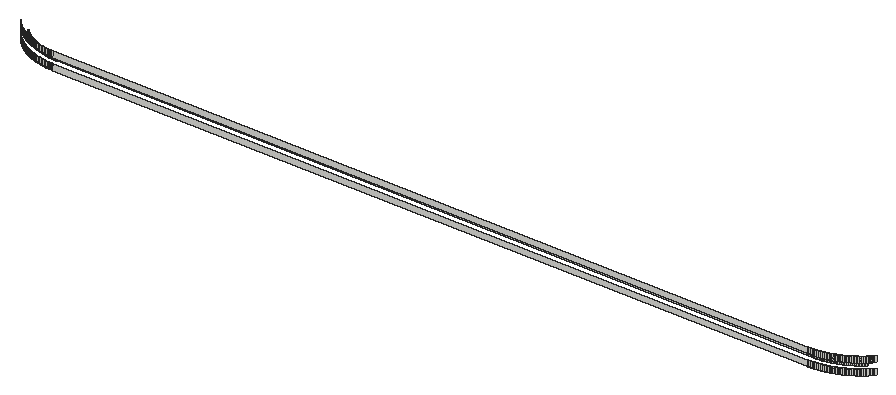
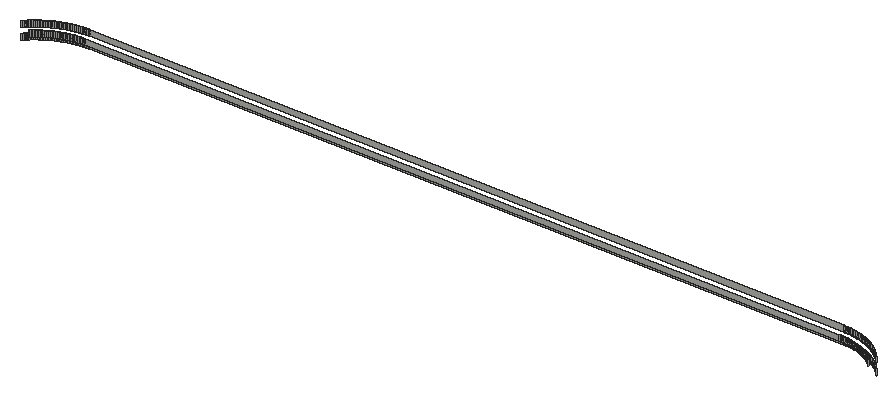
# SketchUp Ruby script. Lengths in inches.
U = 1.inch
M = Sketchup.active_model
def pt(a) = Geom::Point3d.new(a.map { |v| v * U })
def face(e, loops, mat)
  f = e.add_face(loops[0].map { |a| pt(a) })
  loops[1..].each { |l| e.add_face(l.map { |a| pt(a) }).erase! }
  f.material = f.back_material = mat if mat
  f
end
# faces: each face lists its corners as indices into pts; further lists are holes
def faces(e, pts, list, mat = nil) = list.each { |f| face(e, (f[0].is_a?(Array) ? f : [f]).map { |l| l.map { |i| pts[i] } }, mat) }
# xy, xz, yz: faces in a plane at the given z, y or x. An outline is a flat list of corners, or four numbers for a rectangle; further outlines are holes
def ring(l) = l.size == 4 ? [[l[0], l[1]], [l[2], l[1]], [l[2], l[3]], [l[0], l[3]]] : l.each_slice(2).to_a
def flat(e, list, mat, &to3) = list.each { |f| face(e, (f[0].is_a?(Array) ? f : [f]).map { |l| ring(l).map { |u, v| to3.(u, v) } }, mat) }
def xy(e, z, list, mat = nil) = flat(e, list, mat) { |x, y| [x, y, z] }
def xz(e, y, list, mat = nil) = flat(e, list, mat) { |x, z| [x, y, z] }
def yz(e, x, list, mat = nil) = flat(e, list, mat) { |y, z| [x, y, z] }
def lines(e, pts, list) = list.each { |a, b| e.add_line(pt(pts[a]), pt(pts[b])) }
# prism: a flat outline (further loops are holes) pulled along v
def prism(e, loops, v, mat = nil)
  f = face(e, loops, mat); d = Geom::Vector3d.new(v.map { |x| x * U })
  f.pushpull(f.normal.samedirection?(d) ? d.length : -d.length)
end
def box(e, o, s, mat = nil) = prism(e, [[o, [o[0] + s[0], o[1], o[2]], [o[0] + s[0], o[1] + s[1], o[2]], [o[0], o[1] + s[1], o[2]]]], [0, 0, s[2]], mat)
def at(x, y, z, deg = 0) = Geom::Transformation.translation(pt([x, y, z])) * Geom::Transformation.rotation(ORIGIN, Z_AXIS, deg.degrees)
def axes(o, x, y, z) = Geom::Transformation.new([*x, 0, *y, 0, *z, 0, *pt(o).to_a, 1])
def part(name) = M.definitions.add(name)
# library, detail: a bought-in or finely detailed component or shape, given as its bounding box
def library(name, o, s) = part(name).tap { |d| box(d.entities, o, s) }
def detail(e, o, s) = box(e.add_group.entities, o, s)
def put(e, d, t, mat = nil) = e.add_instance(d, t).tap { |i| i.material = mat if mat }
def group(e, t, mat = nil) = e.add_group.tap { |g| g.transformation = t; g.material = mat if mat }.entities
root = M.entities
xz(root,144,[[25.72,392.81,26.03,394.81],[26.03,392.81,290.42,394.81],[290.42,392.81,290.73,394.81],[25.72,396.81,26.03,398.81],[26.03,396.81,290.42,398.81],
  [290.42,396.81,290.73,398.81]])
xz(root,146,[[25.75,394.81,26.04,396.81],[26.04,394.81,290.41,396.81],[290.41,394.81,290.71,396.81]])
p = [[24.46,144.05,392.81],[24.78,144.03,392.81],[24.78,144.03,394.81],[24.46,144.05,394.81],[25.09,144.02,392.81],[25.09,144.02,394.81],
  [25.41,144.01,392.81],[25.41,144.01,394.81],[25.72,144,392.81],[25.72,144,394.81],[290.73,144,392.81],[291.05,144.01,392.81],
  [291.05,144.01,394.81],[290.73,144,394.81],[291.36,144.02,392.81],[291.36,144.02,394.81],[291.68,144.03,392.81],[291.68,144.03,394.81],
  [291.99,144.05,392.81],[291.99,144.05,394.81],[23.21,144.17,392.81],[23.52,144.13,392.81],[23.52,144.13,394.81],[23.21,144.17,394.81],
  [23.84,144.1,392.81],[23.84,144.1,394.81],[24.15,144.07,392.81],[24.15,144.07,394.81],[292.3,144.07,392.81],[292.3,144.07,394.81],
  [292.62,144.1,392.81],[292.62,144.1,394.81],[292.93,144.13,392.81],[292.93,144.13,394.81],[293.24,144.17,392.81],[293.24,144.17,394.81],
  [22.27,144.29,392.81],[22.59,144.25,392.81],[22.59,144.25,394.81],[22.27,144.29,394.81],[22.9,144.2,392.81],[22.9,144.2,394.81],
  [293.56,144.2,392.81],[293.56,144.2,394.81],[293.87,144.25,392.81],[293.87,144.25,394.81],[294.18,144.29,392.81],[294.18,144.29,394.81],
  [21.65,144.4,392.81],[21.96,144.35,392.81],[21.96,144.35,394.81],[21.65,144.4,394.81],[294.49,144.35,392.81],[294.49,144.35,394.81],
  [294.8,144.4,392.81],[294.8,144.4,394.81],[21.35,144.46,392.81],[21.35,144.46,394.81],[295.11,144.46,392.81],[295.11,144.46,394.81],
  [20.73,144.59,392.81],[21.04,144.52,392.81],[21.04,144.52,394.81],[20.73,144.59,394.81],[295.42,144.52,392.81],[295.42,144.52,394.81],
  [295.72,144.59,392.81],[295.72,144.59,394.81],[20.42,144.66,392.81],[20.42,144.66,394.81],[296.03,144.66,392.81],[296.03,144.66,394.81],
  [19.8125,144.82,392.81],[20.12,144.74,392.81],[20.12,144.74,394.81],[19.8125,144.82,394.81],[296.33,144.74,392.81],[296.33,144.74,394.81],
  [296.64,144.82,392.81],[296.64,144.82,394.81],[19.51,144.9,392.81],[19.51,144.9,394.81],[296.94,144.9,392.81],[296.94,144.9,394.81],
  [19.21,144.99,392.81],[19.21,144.99,394.81],[297.24,144.99,392.81],[297.24,144.99,394.81],[18.91,145.08,392.81],[18.91,145.08,394.81],
  [297.55,145.08,392.81],[297.55,145.08,394.81],[18.61,145.17,392.81],[18.61,145.17,394.81],[297.85,145.17,392.81],[297.85,145.17,394.81],
  [18.31,145.27,392.81],[18.31,145.27,394.81],[298.14,145.27,392.81],[298.14,145.27,394.81],[18.01,145.375,392.81],[18.01,145.375,394.81],
  [298.44,145.375,392.81],[298.44,145.375,394.81],[17.72,145.48,392.81],[17.72,145.48,394.81],[298.74,145.48,392.81],[298.74,145.48,394.81],
  [17.42,145.59,392.81],[17.42,145.59,394.81],[299.03,145.59,392.81],[299.03,145.59,394.81],[17.13,145.71,392.81],[17.13,145.71,394.81],
  [299.32,145.71,392.81],[299.32,145.71,394.81],[16.84,145.83,392.81],[16.84,145.83,394.81],[299.62,145.83,392.81],[299.62,145.83,394.81],
  [16.55,145.95,392.81],[16.55,145.95,394.81],[299.91,145.95,392.81],[299.91,145.95,394.81],[16.26,146.07,392.81],[16.26,146.07,394.81],
  [300.19,146.07,392.81],[300.19,146.07,394.81],[15.97,146.2,392.81],[15.97,146.2,394.81],[300.48,146.2,392.81],[300.48,146.2,394.81],
  [15.6875,146.34,392.81],[15.6875,146.34,394.81],[300.77,146.34,392.81],[300.77,146.34,394.81],[15.4,146.47,392.81],[15.4,146.47,394.81],
  [301.05,146.47,392.81],[301.05,146.47,394.81],[15.125,146.61,392.81],[15.125,146.61,394.81],[301.33,146.61,392.81],[301.33,146.61,394.81],
  [14.84,146.76,392.81],[14.84,146.76,394.81],[301.61,146.76,392.81],[301.61,146.76,394.81],[14.57,146.91,392.81],[14.57,146.91,394.81],
  [301.89,146.91,392.81],[301.89,146.91,394.81],[14.29,147.06,392.81],[14.29,147.06,394.81],[302.16,147.06,392.81],[302.16,147.06,394.81],
  [14.02,147.21,392.81],[14.02,147.21,394.81],[302.4375,147.21,392.81],[302.4375,147.21,394.81],[13.75,147.37,392.81],[13.75,147.37,394.81],
  [302.71,147.37,392.81],[302.71,147.37,394.81],[13.48,147.54,392.81],[13.48,147.54,394.81],[302.98,147.54,392.81],[302.98,147.54,394.81],
  [13.21,147.7,392.81],[13.21,147.7,394.81],[303.24,147.7,392.81],[303.24,147.7,394.81],[12.94,147.87,392.81],[12.94,147.87,394.81],
  [303.51,147.87,392.81],[303.51,147.87,394.81],[12.68,148.04,392.81],[12.68,148.04,394.81],[303.77,148.04,392.81],[303.77,148.04,394.81],
  [12.42,148.22,392.81],[12.42,148.22,394.81],[304.03,148.22,392.81],[304.03,148.22,394.81],[12.16,148.4,392.81],[12.16,148.4,394.81],
  [304.29,148.4,392.81],[304.29,148.4,394.81],[11.91,148.58,392.81],[11.91,148.58,394.81],[304.55,148.58,392.81],[304.55,148.58,394.81],
  [11.65,148.77,392.81],[11.65,148.77,394.81],[304.8,148.77,392.81],[304.8,148.77,394.81],[11.4,148.96,392.81],[11.4,148.96,394.81],
  [305.05,148.96,392.81],[305.05,148.96,394.81],[11.16,149.15,392.81],[11.16,149.15,394.81],[305.3,149.15,392.81],[305.3,149.15,394.81],
  [10.91,149.35,392.81],[10.91,149.35,394.81],[305.54,149.35,392.81],[305.54,149.35,394.81],[10.67,149.55,392.81],[10.67,149.55,394.81],
  [305.79,149.55,392.81],[305.79,149.55,394.81],[10.43,149.75,392.81],[10.43,149.75,394.81],[306.03,149.75,392.81],[306.03,149.75,394.81],
  [10.1875,149.95,392.81],[10.1875,149.95,394.81],[306.27,149.95,392.81],[306.27,149.95,394.81],[9.95,150.16,392.81],[9.95,150.16,394.81],
  [306.5,150.16,392.81],[306.5,150.16,394.81],[9.72,150.375,392.81],[9.72,150.375,394.81],[306.73,150.375,392.81],[306.73,150.375,394.81],
  [9.49,150.59,392.81],[9.49,150.59,394.81],[306.96,150.59,392.81],[306.96,150.59,394.81],[9.26,150.81,392.81],[9.26,150.81,394.81],
  [307.19,150.81,392.81],[307.19,150.81,394.81],[9.04,151.03,392.81],[9.04,151.03,394.81],[307.41,151.03,392.81],[307.41,151.03,394.81],
  [8.82,151.25,392.81],[8.82,151.25,394.81],[307.63,151.25,392.81],[307.63,151.25,394.81],[8.6,151.48,392.81],[8.6,151.48,394.81],
  [307.85,151.48,392.81],[307.85,151.48,394.81],[8.39,151.71,392.81],[8.39,151.71,394.81],[308.07,151.71,392.81],[308.07,151.71,394.81],
  [8.17,151.94,392.81],[8.17,151.94,394.81],[308.28,151.94,392.81],[308.28,151.94,394.81],[24.31,146.07,394.81],[24.59,146.05,394.81],
  [24.59,146.05,396.81],[24.31,146.07,396.81],[24.88,146.03,394.81],[24.88,146.03,396.81],[25.17,146.02,394.81],[25.17,146.02,396.81],
  [25.46,146.01,394.81],[25.46,146.01,396.81],[25.75,146,394.81],[25.75,146,396.81],[290.71,146,394.81],[291,146.01,394.81],
  [291,146.01,396.81],[290.71,146,396.81],[291.28,146.02,394.81],[291.28,146.02,396.81],[291.57,146.03,394.81],[291.57,146.03,396.81],
  [291.86,146.05,394.81],[291.86,146.05,396.81],[292.15,146.07,394.81],[292.15,146.07,396.81],[23.44,146.15,394.81],[23.73,146.12,394.81],
  [23.73,146.12,396.81],[23.44,146.15,396.81],[24.02,146.09,394.81],[24.02,146.09,396.81],[292.44,146.09,394.81],[292.44,146.09,396.81],
  [292.72,146.12,394.81],[292.72,146.12,396.81],[293.01,146.15,394.81],[293.01,146.15,396.81],[22.59,146.27,394.81],[22.87,146.23,394.81],
  [22.87,146.23,396.81],[22.59,146.27,396.81],[23.16,146.1875,394.81],[23.16,146.1875,396.81],[293.3,146.1875,394.81],[293.3,146.1875,396.81],
  [293.58,146.23,394.81],[293.58,146.23,396.81],[293.87,146.27,394.81],[293.87,146.27,396.81],[22.02,146.37,394.81],[22.3,146.32,394.81],
  [22.3,146.32,396.81],[22.02,146.37,396.81],[294.15,146.32,394.81],[294.15,146.32,396.81],[294.43,146.37,394.81],[294.43,146.37,396.81],
  [21.45,146.48,394.81],[21.74,146.42,394.81],[21.74,146.42,396.81],[21.45,146.48,396.81],[294.72,146.42,394.81],[294.72,146.42,396.81],
  [295,146.48,394.81],[295,146.48,396.81],[20.89,146.61,394.81],[21.17,146.54,394.81],[21.17,146.54,396.81],[20.89,146.61,396.81],
  [295.28,146.54,394.81],[295.28,146.54,396.81],[295.5625,146.61,394.81],[295.5625,146.61,396.81],[20.61,146.68,394.81],[20.61,146.68,396.81],
  [295.84,146.68,394.81],[295.84,146.68,396.81],[20.05,146.82,394.81],[20.33,146.75,394.81],[20.33,146.75,396.81],[20.05,146.82,396.81],
  [296.12,146.75,394.81],[296.12,146.75,396.81],[296.4,146.82,394.81],[296.4,146.82,396.81],[19.78,146.9,394.81],[19.78,146.9,396.81],
  [296.68,146.9,394.81],[296.68,146.9,396.81],[19.5,146.99,394.81],[19.5,146.99,396.81],[296.95,146.99,394.81],[296.95,146.99,396.81],
  [19.22,147.08,394.81],[19.22,147.08,396.81],[297.23,147.08,394.81],[297.23,147.08,396.81],[18.95,147.17,394.81],[18.95,147.17,396.81],
  [297.5,147.17,394.81],[297.5,147.17,396.81],[18.68,147.26,394.81],[18.68,147.26,396.81],[297.77,147.26,394.81],[297.77,147.26,396.81],
  [18.41,147.36,394.81],[18.41,147.36,396.81],[298.05,147.36,394.81],[298.05,147.36,396.81],[18.14,147.46,394.81],[18.14,147.46,396.81],
  [298.32,147.46,394.81],[298.32,147.46,396.81],[17.87,147.57,394.81],[17.87,147.57,396.81],[298.58,147.57,394.81],[298.58,147.57,396.81],
  [17.6,147.67,394.81],[17.6,147.67,396.81],[298.85,147.67,394.81],[298.85,147.67,396.81],[17.34,147.79,394.81],[17.34,147.79,396.81],
  [299.12,147.79,394.81],[299.12,147.79,396.81],[17.07,147.9,394.81],[17.07,147.9,396.81],[299.38,147.9,394.81],[299.38,147.9,396.81],
  [16.81,148.02,394.81],[16.81,148.02,396.81],[299.64,148.02,394.81],[299.64,148.02,396.81],[16.55,148.14,394.81],[16.55,148.14,396.81],
  [299.91,148.14,394.81],[299.91,148.14,396.81],[16.29,148.27,394.81],[16.29,148.27,396.81],[300.17,148.27,394.81],[300.17,148.27,396.81],
  [16.03,148.4,394.81],[16.03,148.4,396.81],[300.42,148.4,394.81],[300.42,148.4,396.81],[15.77,148.53,394.81],[15.77,148.53,396.81],
  [300.68,148.53,394.81],[300.68,148.53,396.81],[15.52,148.67,394.81],[15.52,148.67,396.81],[300.93,148.67,394.81],[300.93,148.67,396.81],
  [15.27,148.8,394.81],[15.27,148.8,396.81],[301.1875,148.8,394.81],[301.1875,148.8,396.81],[15.02,148.95,394.81],[15.02,148.95,396.81],
  [301.4375,148.95,394.81],[301.4375,148.95,396.81],[14.77,149.09,394.81],[14.77,149.09,396.81],[301.6875,149.09,394.81],[301.6875,149.09,396.81],
  [14.52,149.24,394.81],[14.52,149.24,396.81],[301.93,149.24,394.81],[301.93,149.24,396.81],[14.28,149.39,394.81],[14.28,149.39,396.81],
  [302.18,149.39,394.81],[302.18,149.39,396.81],[14.03,149.55,394.81],[14.03,149.55,396.81],[302.42,149.55,394.81],[302.42,149.55,396.81],
  [13.79,149.71,394.81],[13.79,149.71,396.81],[302.66,149.71,394.81],[302.66,149.71,396.81],[13.55,149.87,394.81],[13.55,149.87,396.81],
  [302.9,149.87,394.81],[302.9,149.87,396.81],[13.32,150.03,394.81],[13.32,150.03,396.81],[303.14,150.03,394.81],[303.14,150.03,396.81],
  [13.08,150.2,394.81],[13.08,150.2,396.81],[303.37,150.2,394.81],[303.37,150.2,396.81],[12.85,150.37,394.81],[12.85,150.37,396.81],
  [303.6,150.37,394.81],[303.6,150.37,396.81],[12.62,150.55,394.81],[12.62,150.55,396.81],[303.83,150.55,394.81],[303.83,150.55,396.81],
  [12.39,150.72,394.81],[12.39,150.72,396.81],[304.0625,150.72,394.81],[304.0625,150.72,396.81],[12.17,150.9,394.81],[12.17,150.9,396.81],
  [304.29,150.9,394.81],[304.29,150.9,396.81],[11.94,151.09,394.81],[11.94,151.09,396.81],[304.51,151.09,394.81],[304.51,151.09,396.81],
  [11.72,151.27,394.81],[11.72,151.27,396.81],[304.73,151.27,394.81],[304.73,151.27,396.81],[11.51,151.46,394.81],[11.51,151.46,396.81],
  [304.95,151.46,394.81],[304.95,151.46,396.81],[11.29,151.65,394.81],[11.29,151.65,396.81],[305.16,151.65,394.81],[305.16,151.65,396.81],
  [11.08,151.84,394.81],[11.08,151.84,396.81],[305.375,151.84,394.81],[305.375,151.84,396.81],[10.87,152.04,394.81],[10.87,152.04,396.81],
  [24.46,144.05,396.81],[24.78,144.03,396.81],[24.78,144.03,398.81],[24.46,144.05,398.81],[25.09,144.02,396.81],[25.09,144.02,398.81],
  [25.41,144.01,396.81],[25.41,144.01,398.81],[25.72,144,396.81],[25.72,144,398.81],[290.73,144,396.81],[291.05,144.01,396.81],
  [291.05,144.01,398.81],[290.73,144,398.81],[291.36,144.02,396.81],[291.36,144.02,398.81],[291.68,144.03,396.81],[291.68,144.03,398.81],
  [291.99,144.05,396.81],[291.99,144.05,398.81],[23.21,144.17,396.81],[23.52,144.13,396.81],[23.52,144.13,398.81],[23.21,144.17,398.81],
  [23.84,144.1,396.81],[23.84,144.1,398.81],[24.15,144.07,396.81],[24.15,144.07,398.81],[292.3,144.07,396.81],[292.3,144.07,398.81],
  [292.62,144.1,396.81],[292.62,144.1,398.81],[292.93,144.13,396.81],[292.93,144.13,398.81],[293.24,144.17,396.81],[293.24,144.17,398.81],
  [22.27,144.29,396.81],[22.59,144.25,396.81],[22.59,144.25,398.81],[22.27,144.29,398.81],[22.9,144.2,396.81],[22.9,144.2,398.81],
  [293.56,144.2,396.81],[293.56,144.2,398.81],[293.87,144.25,396.81],[293.87,144.25,398.81],[294.18,144.29,396.81],[294.18,144.29,398.81],
  [21.65,144.4,396.81],[21.96,144.35,396.81],[21.96,144.35,398.81],[21.65,144.4,398.81],[294.49,144.35,396.81],[294.49,144.35,398.81],
  [294.8,144.4,396.81],[294.8,144.4,398.81],[21.35,144.46,396.81],[21.35,144.46,398.81],[295.11,144.46,396.81],[295.11,144.46,398.81],
  [20.73,144.59,396.81],[21.04,144.52,396.81],[21.04,144.52,398.81],[20.73,144.59,398.81],[295.42,144.52,396.81],[295.42,144.52,398.81],
  [295.72,144.59,396.81],[295.72,144.59,398.81],[20.42,144.66,396.81],[20.42,144.66,398.81],[296.03,144.66,396.81],[296.03,144.66,398.81],
  [19.8125,144.82,396.81],[20.12,144.74,396.81],[20.12,144.74,398.81],[19.8125,144.82,398.81],[296.33,144.74,396.81],[296.33,144.74,398.81],
  [296.64,144.82,396.81],[296.64,144.82,398.81],[19.51,144.9,396.81],[19.51,144.9,398.81],[296.94,144.9,396.81],[296.94,144.9,398.81],
  [19.21,144.99,396.81],[19.21,144.99,398.81],[297.24,144.99,396.81],[297.24,144.99,398.81],[18.91,145.08,396.81],[18.91,145.08,398.81],
  [297.55,145.08,396.81],[297.55,145.08,398.81],[18.61,145.17,396.81],[18.61,145.17,398.81],[297.85,145.17,396.81],[297.85,145.17,398.81],
  [18.31,145.27,396.81],[18.31,145.27,398.81],[298.14,145.27,396.81],[298.14,145.27,398.81],[18.01,145.375,396.81],[18.01,145.375,398.81],
  [298.44,145.375,396.81],[298.44,145.375,398.81],[17.72,145.48,396.81],[17.72,145.48,398.81],[298.74,145.48,396.81],[298.74,145.48,398.81],
  [17.42,145.59,396.81],[17.42,145.59,398.81],[299.03,145.59,396.81],[299.03,145.59,398.81],[17.13,145.71,396.81],[17.13,145.71,398.81],
  [299.32,145.71,396.81],[299.32,145.71,398.81],[16.84,145.83,396.81],[16.84,145.83,398.81],[299.62,145.83,396.81],[299.62,145.83,398.81],
  [16.55,145.95,396.81],[16.55,145.95,398.81],[299.91,145.95,396.81],[299.91,145.95,398.81],[16.26,146.07,396.81],[16.26,146.07,398.81],
  [300.19,146.07,396.81],[300.19,146.07,398.81],[15.97,146.2,396.81],[15.97,146.2,398.81],[300.48,146.2,396.81],[300.48,146.2,398.81],
  [15.6875,146.34,396.81],[15.6875,146.34,398.81],[300.77,146.34,396.81],[300.77,146.34,398.81],[15.4,146.47,396.81],[15.4,146.47,398.81],
  [301.05,146.47,396.81],[301.05,146.47,398.81],[15.125,146.61,396.81],[15.125,146.61,398.81],[301.33,146.61,396.81],[301.33,146.61,398.81],
  [14.84,146.76,396.81],[14.84,146.76,398.81],[301.61,146.76,396.81],[301.61,146.76,398.81],[14.57,146.91,396.81],[14.57,146.91,398.81],
  [301.89,146.91,396.81],[301.89,146.91,398.81],[14.29,147.06,396.81],[14.29,147.06,398.81],[302.16,147.06,396.81],[302.16,147.06,398.81],
  [14.02,147.21,396.81],[14.02,147.21,398.81],[302.4375,147.21,396.81],[302.4375,147.21,398.81],[13.75,147.37,396.81],[13.75,147.37,398.81],
  [302.71,147.37,396.81],[302.71,147.37,398.81],[13.48,147.54,396.81],[13.48,147.54,398.81],[302.98,147.54,396.81],[302.98,147.54,398.81],
  [13.21,147.7,396.81],[13.21,147.7,398.81],[303.24,147.7,396.81],[303.24,147.7,398.81],[12.94,147.87,396.81],[12.94,147.87,398.81],
  [303.51,147.87,396.81],[303.51,147.87,398.81],[12.68,148.04,396.81],[12.68,148.04,398.81],[303.77,148.04,396.81],[303.77,148.04,398.81],
  [12.42,148.22,396.81],[12.42,148.22,398.81],[304.03,148.22,396.81],[304.03,148.22,398.81],[12.16,148.4,396.81],[12.16,148.4,398.81],
  [304.29,148.4,396.81],[304.29,148.4,398.81],[11.91,148.58,396.81],[11.91,148.58,398.81],[304.55,148.58,396.81],[304.55,148.58,398.81],
  [11.65,148.77,396.81],[11.65,148.77,398.81],[304.8,148.77,396.81],[304.8,148.77,398.81],[11.4,148.96,396.81],[11.4,148.96,398.81],
  [305.05,148.96,396.81],[305.05,148.96,398.81],[11.16,149.15,396.81],[11.16,149.15,398.81],[305.3,149.15,396.81],[305.3,149.15,398.81],
  [10.91,149.35,396.81],[10.91,149.35,398.81],[305.54,149.35,396.81],[305.54,149.35,398.81],[10.67,149.55,396.81],[10.67,149.55,398.81],
  [305.79,149.55,396.81],[305.79,149.55,398.81],[10.43,149.75,396.81],[10.43,149.75,398.81],[306.03,149.75,396.81],[306.03,149.75,398.81],
  [10.1875,149.95,396.81],[10.1875,149.95,398.81],[306.27,149.95,396.81],[306.27,149.95,398.81],[9.95,150.16,396.81],[9.95,150.16,398.81],
  [306.5,150.16,396.81],[306.5,150.16,398.81],[9.72,150.375,396.81],[9.72,150.375,398.81],[306.73,150.375,396.81],[306.73,150.375,398.81],
  [9.49,150.59,396.81],[9.49,150.59,398.81],[306.96,150.59,396.81],[306.96,150.59,398.81],[9.26,150.81,396.81],[9.26,150.81,398.81],
  [307.19,150.81,396.81],[307.19,150.81,398.81],[9.04,151.03,396.81],[9.04,151.03,398.81],[307.41,151.03,396.81],[307.41,151.03,398.81],
  [8.82,151.25,396.81],[8.82,151.25,398.81],[307.63,151.25,396.81],[307.63,151.25,398.81],[8.6,151.48,396.81],[8.6,151.48,398.81],
  [307.85,151.48,396.81],[307.85,151.48,398.81],[8.39,151.71,396.81],[8.39,151.71,398.81],[308.07,151.71,396.81],[308.07,151.71,398.81],
  [8.17,151.94,396.81],[8.17,151.94,398.81],[308.28,151.94,396.81],[308.28,151.94,398.81],[26.04,146,396.81],[26.04,146,398.81],
  [290.41,146,396.81],[290.41,146,398.81]]
faces(root,p,[[0,1,2,3],[1,4,5,2],[4,6,7,5],[6,8,9,7],[10,11,12,13],[11,14,15,12],[14,16,17,15],[16,18,19,17],
  [20,21,22,23],[21,24,25,22],[24,26,27,25],[26,0,3,27],[18,28,29,19],[28,30,31,29],[30,32,33,31],[32,34,35,33],
  [36,37,38,39],[37,40,41,38],[40,20,23,41],[34,42,43,35],[42,44,45,43],[44,46,47,45],[48,49,50,51],[49,36,39,50],
  [46,52,53,47],[52,54,55,53],[56,48,51,57],[54,58,59,55],[60,61,62,63],[61,56,57,62],[58,64,65,59],[64,66,67,65],
  [68,60,63,69],[66,70,71,67],[72,73,74,75],[73,68,69,74],[70,76,77,71],[76,78,79,77],[80,72,75,81],[78,82,83,79],
  [84,80,81,85],[82,86,87,83],[88,84,85,89],[86,90,91,87],[92,88,89,93],[90,94,95,91],[96,92,93,97],[94,98,99,95],
  [100,96,97,101],[98,102,103,99],[104,100,101,105],[102,106,107,103],[108,104,105,109],[106,110,111,107],[112,108,109,113],[110,114,115,111],
  [116,112,113,117],[114,118,119,115],[120,116,117,121],[118,122,123,119],[124,120,121,125],[122,126,127,123],[128,124,125,129],[126,130,131,127],
  [132,128,129,133],[130,134,135,131],[136,132,133,137],[134,138,139,135],[140,136,137,141],[138,142,143,139],[144,140,141,145],[142,146,147,143],
  [148,144,145,149],[146,150,151,147],[152,148,149,153],[150,154,155,151],[156,152,153,157],[154,158,159,155],[160,156,157,161],[158,162,163,159],
  [164,160,161,165],[162,166,167,163],[168,164,165,169],[166,170,171,167],[172,168,169,173],[170,174,175,171],[176,172,173,177],[174,178,179,175],
  [180,176,177,181],[178,182,183,179],[184,180,181,185],[182,186,187,183],[188,184,185,189],[186,190,191,187],[192,188,189,193],[190,194,195,191],
  [196,192,193,197],[194,198,199,195],[200,196,197,201],[198,202,203,199],[204,200,201,205],[202,206,207,203],[208,204,205,209],[206,210,211,207],
  [212,208,209,213],[210,214,215,211],[216,212,213,217],[214,218,219,215],[220,216,217,221],[218,222,223,219],[224,220,221,225],[222,226,227,223],
  [228,224,225,229],[226,230,231,227],[232,228,229,233],[230,234,235,231],[236,232,233,237],[234,238,239,235],[240,236,237,241],[238,242,243,239],
  [244,240,241,245],[242,246,247,243],[248,244,245,249],[246,250,251,247],[252,248,249,253],[250,254,255,251],[256,257,258,259],[257,260,261,258],
  [260,262,263,261],[262,264,265,263],[264,266,267,265],[268,269,270,271],[269,272,273,270],[272,274,275,273],[274,276,277,275],[276,278,279,277],
  [280,281,282,283],[281,284,285,282],[284,256,259,285],[278,286,287,279],[286,288,289,287],[288,290,291,289],[292,293,294,295],[293,296,297,294],
  [296,280,283,297],[290,298,299,291],[298,300,301,299],[300,302,303,301],[304,305,306,307],[305,292,295,306],[302,308,309,303],[308,310,311,309],
  [312,313,314,315],[313,304,307,314],[310,316,317,311],[316,318,319,317],[320,321,322,323],[321,312,315,322],[318,324,325,319],[324,326,327,325],
  [328,320,323,329],[326,330,331,327],[332,333,334,335],[333,328,329,334],[330,336,337,331],[336,338,339,337],[340,332,335,341],[338,342,343,339],
  [344,340,341,345],[342,346,347,343],[348,344,345,349],[346,350,351,347],[352,348,349,353],[350,354,355,351],[356,352,353,357],[354,358,359,355],
  [360,356,357,361],[358,362,363,359],[364,360,361,365],[362,366,367,363],[368,364,365,369],[366,370,371,367],[372,368,369,373],[370,374,375,371],
  [376,372,373,377],[374,378,379,375],[380,376,377,381],[378,382,383,379],[384,380,381,385],[382,386,387,383],[388,384,385,389],[386,390,391,387],
  [392,388,389,393],[390,394,395,391],[396,392,393,397],[394,398,399,395],[400,396,397,401],[398,402,403,399],[404,400,401,405],[402,406,407,403],
  [408,404,405,409],[406,410,411,407],[412,408,409,413],[410,414,415,411],[416,412,413,417],[414,418,419,415],[420,416,417,421],[418,422,423,419],
  [424,420,421,425],[422,426,427,423],[428,424,425,429],[426,430,431,427],[432,428,429,433],[430,434,435,431],[436,432,433,437],[434,438,439,435],
  [440,436,437,441],[438,442,443,439],[444,440,441,445],[442,446,447,443],[448,444,445,449],[446,450,451,447],[452,448,449,453],[450,454,455,451],
  [456,452,453,457],[454,458,459,455],[460,456,457,461],[458,462,463,459],[464,460,461,465],[462,466,467,463],[468,464,465,469],[466,470,471,467],
  [472,468,469,473],[470,474,475,471],[476,472,473,477],[474,478,479,475],[480,476,477,481],[478,482,483,479],[484,480,481,485],[486,487,488,489],
  [487,490,491,488],[490,492,493,491],[492,494,495,493],[496,497,498,499],[497,500,501,498],[500,502,503,501],[502,504,505,503],[506,507,508,509],
  [507,510,511,508],[510,512,513,511],[512,486,489,513],[504,514,515,505],[514,516,517,515],[516,518,519,517],[518,520,521,519],[522,523,524,525],
  [523,526,527,524],[526,506,509,527],[520,528,529,521],[528,530,531,529],[530,532,533,531],[534,535,536,537],[535,522,525,536],[532,538,539,533],
  [538,540,541,539],[542,534,537,543],[540,544,545,541],[546,547,548,549],[547,542,543,548],[544,550,551,545],[550,552,553,551],[554,546,549,555],
  [552,556,557,553],[558,559,560,561],[559,554,555,560],[556,562,563,557],[562,564,565,563],[566,558,561,567],[564,568,569,565],[570,566,567,571],
  [568,572,573,569],[574,570,571,575],[572,576,577,573],[578,574,575,579],[576,580,581,577],[582,578,579,583],[580,584,585,581],[586,582,583,587],
  [584,588,589,585],[590,586,587,591],[588,592,593,589],[594,590,591,595],[592,596,597,593],[598,594,595,599],[596,600,601,597],[602,598,599,603],
  [600,604,605,601],[606,602,603,607],[604,608,609,605],[610,606,607,611],[608,612,613,609],[614,610,611,615],[612,616,617,613],[618,614,615,619],
  [616,620,621,617],[622,618,619,623],[620,624,625,621],[626,622,623,627],[624,628,629,625],[630,626,627,631],[628,632,633,629],[634,630,631,635],
  [632,636,637,633],[638,634,635,639],[636,640,641,637],[642,638,639,643],[640,644,645,641],[646,642,643,647],[644,648,649,645],[650,646,647,651],
  [648,652,653,649],[654,650,651,655],[652,656,657,653],[658,654,655,659],[656,660,661,657],[662,658,659,663],[660,664,665,661],[666,662,663,667],
  [664,668,669,665],[670,666,667,671],[668,672,673,669],[674,670,671,675],[672,676,677,673],[678,674,675,679],[676,680,681,677],[682,678,679,683],
  [680,684,685,681],[686,682,683,687],[684,688,689,685],[690,686,687,691],[688,692,693,689],[694,690,691,695],[692,696,697,693],[698,694,695,699],
  [696,700,701,697],[702,698,699,703],[700,704,705,701],[706,702,703,707],[704,708,709,705],[710,706,707,711],[708,712,713,709],[714,710,711,715],
  [712,716,717,713],[718,714,715,719],[716,720,721,717],[722,718,719,723],[720,724,725,721],[726,722,723,727],[724,728,729,725],[730,726,727,731],
  [728,732,733,729],[734,730,731,735],[732,736,737,733],[738,734,735,739],[736,740,741,737]])
lines(root,p,[[742,743],[744,745]])
